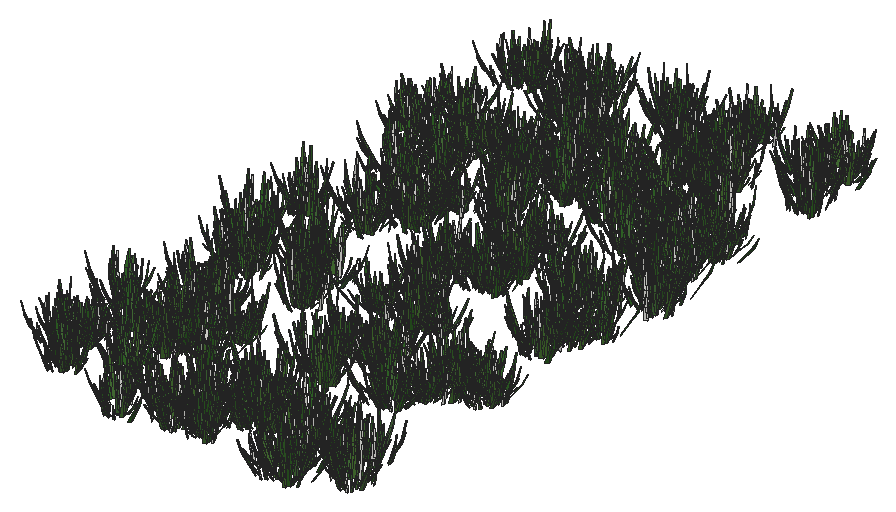
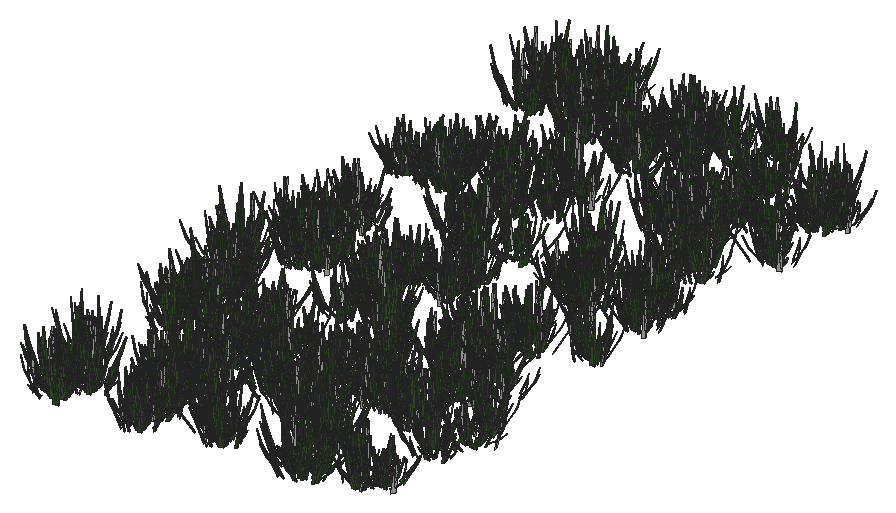
# SketchUp Ruby script. Lengths in inches.
U = 1.inch
M = Sketchup.active_model
def pt(a) = Geom::Point3d.new(a.map { |v| v * U })
def face(e, loops, mat)
  f = e.add_face(loops[0].map { |a| pt(a) })
  loops[1..].each { |l| e.add_face(l.map { |a| pt(a) }).erase! }
  f.material = f.back_material = mat if mat
  f
end
# faces: each face lists its corners as indices into pts; further lists are holes
def faces(e, pts, list, mat = nil) = list.each { |f| face(e, (f[0].is_a?(Array) ? f : [f]).map { |l| l.map { |i| pts[i] } }, mat) }
# xy, xz, yz: faces in a plane at the given z, y or x. An outline is a flat list of corners, or four numbers for a rectangle; further outlines are holes
def ring(l) = l.size == 4 ? [[l[0], l[1]], [l[2], l[1]], [l[2], l[3]], [l[0], l[3]]] : l.each_slice(2).to_a
def flat(e, list, mat, &to3) = list.each { |f| face(e, (f[0].is_a?(Array) ? f : [f]).map { |l| ring(l).map { |u, v| to3.(u, v) } }, mat) }
def xy(e, z, list, mat = nil) = flat(e, list, mat) { |x, y| [x, y, z] }
def xz(e, y, list, mat = nil) = flat(e, list, mat) { |x, z| [x, y, z] }
def yz(e, x, list, mat = nil) = flat(e, list, mat) { |y, z| [x, y, z] }
def lines(e, pts, list) = list.each { |a, b| e.add_line(pt(pts[a]), pt(pts[b])) }
# prism: a flat outline (further loops are holes) pulled along v
def prism(e, loops, v, mat = nil)
  f = face(e, loops, mat); d = Geom::Vector3d.new(v.map { |x| x * U })
  f.pushpull(f.normal.samedirection?(d) ? d.length : -d.length)
end
def box(e, o, s, mat = nil) = prism(e, [[o, [o[0] + s[0], o[1], o[2]], [o[0] + s[0], o[1] + s[1], o[2]], [o[0], o[1] + s[1], o[2]]]], [0, 0, s[2]], mat)
def at(x, y, z, deg = 0) = Geom::Transformation.translation(pt([x, y, z])) * Geom::Transformation.rotation(ORIGIN, Z_AXIS, deg.degrees)
def axes(o, x, y, z) = Geom::Transformation.new([*x, 0, *y, 0, *z, 0, *pt(o).to_a, 1])
def part(name) = M.definitions.add(name)
# library, detail: a bought-in or finely detailed component or shape, given as its bounding box
def library(name, o, s) = part(name).tap { |d| box(d.entities, o, s) }
def detail(e, o, s) = box(e.add_group.entities, o, s)
def put(e, d, t, mat = nil) = e.add_instance(d, t).tap { |i| i.material = mat if mat }
def group(e, t, mat = nil) = e.add_group.tap { |g| g.transformation = t; g.material = mat if mat }.entities
root = M.entities
M.materials.add("Material1").color = [58, 110, 58]
M.materials.add("Material10").color = [48, 100, 38]
M.materials.add("Material3").color = [68, 110, 58]
M.materials.add("Material4").color = [48, 90, 38]
M.materials.add("Material5").color = [68, 110, 48]
M.materials.add("Material6").color = [48, 90, 48]
M.materials.add("Material8").color = [58, 90, 38]
M.materials.add("Material9").color = [68, 100, 58]
c1 = part("grass00")
p = [[-0.6875,0.15,0],[-0.56,0.08,5.52],[-0.04,0.03,2.76],[0.48,-0.02,0],[0.35,-0.02,5.52],[-0.1,-0.14,5.52],
  [-0.12,0.65,8.37],[-0.42,0.65,8.37]]
faces(c1.entities,p,[[0,1,2,3],[3,2,4],[1,5,2],[5,4,2],[1,6,5],[4,5,6],[7,6,1]])
c2 = part("Group16\#1")
put(c2.entities,c1,axes([1.44,-0.61,-0.01],[0.05352,0.12609,0],[-0.10704,0.04543,0.07239],[0.06664,-0.02828,0.11628]),"Material6")
put(c2.entities,c1,axes([0.76,-0.15,-0.01],[0.04676,0.24062,0],[-0.23162,0.04501,0.06642],[0.0652,-0.01267,0.23595]),"Material3")
put(c2.entities,c1,axes([0.79,0.01,-0.01],[-0.00606,0.34651,0],[-0.34381,-0.00602,0.0432],[0.04319,0.00076,0.34386]))
put(c2.entities,c1,axes([1,0.23,-0.01],[-0.07192,0.31144,0],[-0.28722,-0.06632,0.1236],[0.12043,0.02781,0.29478]),"Material5")
put(c2.entities,c1,axes([1.66,0.77,-0.01],[-0.13828,0.29651,0],[-0.21551,-0.1005,0.22471],[0.20365,0.09498,0.23779]),"Material10")
put(c2.entities,c1,axes([0.6875,0.52,-0.01],[-0.18126,0.24051,0],[-0.22746,-0.17142,0.09788],[0.07817,0.05891,0.28481]),"Material5")
put(c2.entities,c1,axes([0.68,0.78,-0.01],[-0.215,0.18688,0],[-0.12385,-0.14248,0.21334],[0.13995,0.16101,0.18878]),"Material3")
put(c2.entities,c1,axes([0.56,1,-0.01],[-0.13756,0.07624,0],[-0.06159,-0.11112,0.0927],[0.04494,0.08108,0.12705]),"Material5")
put(c2.entities,c1,axes([0.2,0.64,-0.01],[-0.23729,0.07254,0],[-0.05711,-0.18681,0.153],[0.04473,0.14632,0.19535]),"Material10")
put(c2.entities,c1,axes([0.0625,0.72,-0.01],[-0.28874,0.02525,0],[-0.02179,-0.24916,0.14647],[0.01276,0.14591,0.25012]),"Material3")
put(c2.entities,c1,axes([-0.08,0.62,-0.01],[-0.34089,-0.04187,0],[0.03255,-0.26504,0.216],[-0.02633,0.21439,0.26703]),"Material10")
put(c2.entities,c1,axes([-0.34,0.98,-0.01],[-0.14314,-0.0493,0],[0.04397,-0.12769,0.06843],[-0.02228,0.0647,0.13505]),"Material10")
put(c2.entities,c1,axes([-0.87,1.45,-0.01],[-0.23488,-0.14114,0],[0.13761,-0.22901,0.06087],[-0.03135,0.05217,0.26717]))
put(c2.entities,c1,axes([-0.72,0.77,-0.01],[-0.14208,-0.13251,0],[0.07209,-0.0773,0.16301],[-0.11118,0.11922,0.1057]),"Material10")
put(c2.entities,c1,axes([-0.62,0.43,-0.01],[-0.14845,-0.21203,0],[0.18654,-0.13061,0.12304],[-0.10079,0.07057,0.22772]),"Material3")
put(c2.entities,c1,axes([-0.68,0.29,-0.01],[-0.13639,-0.32136,0],[0.31723,-0.13464,0.05579],[-0.05136,0.0218,0.34462]),"Material4")
put(c2.entities,c1,axes([-0.64,0.125,-0.01],[-0.0458,-0.23569,0],[0.22124,-0.043,0.08276],[-0.08124,0.01579,0.22538]),"Material1")
put(c2.entities,c1,axes([-1.6,-0.03,-0.01],[0.00576,-0.32897,0],[0.27526,0.00482,0.18018],[-0.18015,-0.00315,0.2753]),"Material5")
put(c2.entities,c1,axes([-1.36,-0.31,-0.01],[0.05718,-0.24765,0],[0.18172,0.04196,0.17267],[-0.16825,-0.03885,0.1865]),"Material10")
put(c2.entities,c1,axes([-1.54,-0.72,-0.01],[0.06537,-0.14017,0],[0.13555,0.06321,0.03939],[-0.0357,-0.01665,0.14956]))
put(c2.entities,c1,axes([-1.19,-0.9,-0.01],[0.09597,-0.12735,0],[0.11214,0.08451,0.07557],[-0.06035,-0.04548,0.14042]),"Material9")
put(c2.entities,c1,axes([-0.47,-0.54,-0.01],[0.11588,-0.10072,0],[0.0618,0.0711,0.12124],[-0.07953,-0.0915,0.0942]))
put(c2.entities,c1,axes([-0.47,-0.84,-0.01],[0.11927,-0.0661,0],[0.06603,0.11913,0.00646],[-0.00313,-0.00565,0.13621]),"Material5")
put(c2.entities,c1,axes([-0.38,-1.24,-0.01],[0.28037,-0.08571,0],[0.0618,0.20215,0.20315],[-0.05939,-0.19428,0.21139]),"Material9")
put(c2.entities,c1,axes([-0.06,-0.66,-0.01],[0.22719,-0.01987,0],[0.01247,0.14255,0.17758],[-0.01547,-0.17691,0.1431]),"Material8")
put(c2.entities,c1,axes([0.11,-0.89,-0.01],[0.14882,0.01828,0],[-0.01058,0.08611,0.12229],[0.01491,-0.12138,0.08676]),"Material6")
put(c2.entities,c1,axes([0.25,-0.72,-0.01],[0.20481,0.07053,0],[-0.06206,0.18022,0.10291],[0.03351,-0.0973,0.1906]),"Material6")
put(c2.entities,c1,axes([0.85,-1.42,-0.01],[0.16481,0.09904,0],[-0.09472,0.15762,0.05616],[0.02893,-0.04814,0.18389]),"Material5")
put(c2.entities,c1,axes([1.01,-1.09,-0.01],[0.21858,0.20385,0],[-0.17495,0.1876,0.15339],[0.10462,-0.11218,0.25652]),"Material10")
put(c2.entities,c1,axes([1.01,-0.71,-0.01],[0.08733,0.12473,0],[-0.06445,0.04512,0.13037],[0.1068,-0.07477,0.07867]),"Material6")
c3 = part("Group15\#1")
put(c3.entities,c2,at(0,0,0))
c4 = part("3darcstudiotree_grass00\#1")
put(c4.entities,c3,at(0,0,0))
put(root,c4,axes([299.44,103.05,0.25],[0.93913,0.57202,0],[-0.54019,0.61097,-0.01519],[-0.01329,0.01503,1.34969]))
put(root,c4,axes([299.53,110.64,0.25],[1.10058,0.261,0],[-0.28805,0.83679,-0.01128],[-0.00476,0.01382,1.61003]))
put(root,c4,axes([300.52,104.49,0.25],[-0.9392,-0.54137,0],[0.54982,-0.65712,-0.00375],[0.00405,-0.00484,1.82358]))
put(root,c4,axes([299.93,147.66,0.25],[0.46431,0.89389,0],[-1.16621,0.41731,-0.01792],[-0.01737,0.00622,1.34035]))
put(root,c4,axes([300.54,144.8125,0.25],[0.73834,-0.68186,0],[0.67706,0.50505,-0.01288],[0.01631,0.01217,1.54961]))
put(root,c4,axes([300.53,103.35,0.25],[0.71679,0.74501,0],[-0.71323,0.47274,-0.01421],[-0.01715,0.01137,1.40932]))
put(root,c4,axes([301.02,122.21,0.25],[-0.0646,-0.98333,0],[0.90905,-0.04114,-0.01049],[0.0169,-0.00076,1.4693]))
put(root,c4,axes([301.24,151.2,0.25],[-0.89627,-0.50604,0],[0.648,-0.79066,-0.01911],[0.01239,-0.01512,1.32815]))
put(root,c4,axes([301.26,131.3,0.25],[0.71286,-0.77446,0],[0.82334,0.52208,-0.00592],[0.00812,0.00515,1.78738]))
put(root,c4,axes([301.23,125.5,0.25],[1.11911,0.29462,0],[-0.34141,0.8934,-0.00141],[-0.00074,0.00193,1.95289]))
put(root,c4,axes([301.5,157.36,0.25],[1.00744,0.57948,0],[-0.6913,0.82795,-0.01195],[-0.00771,0.00924,1.37528]))
put(root,c4,axes([302.64,116.1,0.25],[-0.51912,-0.87799,0],[1.01268,-0.41248,-0.01008],[0.01256,-0.00511,1.566]))
put(root,c4,axes([302.18,99.9375,0.25],[0.69262,0.55781,0],[-0.64459,0.55138,-0.00683],[-0.00897,0.00768,1.74693]))
put(root,c4,axes([302.68,158.2,0.25],[0.15903,-0.85053,0],[0.92507,0.11916,-0.00401],[0.00771,0.00099,1.82024]))
put(root,c4,axes([302.75,122.15,0.25],[-0.79135,0.83075,0],[-0.79545,-0.52199,-0.0043],[-0.00623,-0.00409,1.8735]))
put(root,c4,axes([302.81,107.06,0.25],[0.98585,0.35764,0],[-0.42278,0.80286,-0.01451],[-0.00881,0.01673,1.59989]))
put(root,c4,axes([303.12,140.61,0.25],[1.26422,0.21833,0],[-0.2641,1.05349,-0.01168],[-0.00256,0.01022,1.39591]))
put(root,c4,axes([303.91,120.59,0.25],[0.5832,0.63351,0],[-0.84564,0.53629,-0.0123],[-0.01469,0.00931,1.59876]))
put(root,c4,axes([305.61,148.46,0.25],[-0.29231,-0.74071,0],[1.21148,-0.32935,-0.01545],[0.01785,-0.00485,1.54954]))
put(root,c4,axes([305.17,111.68,0.25],[-0.10149,1.06077,0],[-1.17045,-0.07715,-0.01448],[-0.01792,-0.00118,1.45727]))
put(root,c4,axes([305.58,133.39,0.25],[-1.00175,0.10113,0],[-0.15478,-1.05623,-0.00408],[-0.00067,-0.00459,1.74968]))
put(root,c4,axes([305.25,146.88,0.25],[-0.29516,0.99433,0],[-1.18202,-0.24172,-0.00818],[-0.0119,-0.00243,1.82396]))
put(root,c4,axes([305.51,143.13,0.25],[0.81075,0.69136,0],[-0.85148,0.68788,-0.004],[-0.00456,0.00369,1.89371]))
put(root,c4,axes([306,137.53,0.25],[-1.13548,0.14887,0],[-0.16361,-0.85972,-0.01239],[-0.00262,-0.01379,1.42361]))
put(root,c4,axes([305.7,115.38,0.25],[-0.33676,0.92684,0],[-1.01936,-0.25516,-0.01363],[-0.01733,-0.00434,1.41312]))
put(root,c4,axes([306.17,125.84,0.25],[0.94821,0.33617,0],[-0.44135,0.85759,-0.00364],[-0.00249,0.00485,1.96053]))
put(root,c4,axes([306.94,124.85,0.25],[-0.71892,-0.83603,0],[0.93762,-0.55545,-0.01802],[0.01713,-0.01015,1.345]))
put(root,c4,axes([306.99,160.35,0.25],[-1.10649,-0.54201,0],[0.48134,-0.67694,-0.01139],[0.00932,-0.01311,1.52439]))
put(root,c4,axes([306.61,107.01,0.25],[-0.5773,0.77336,0],[-0.97603,-0.50192,-0.01218],[-0.0144,-0.0074,1.59607]))
put(root,c4,axes([307.02,132.05,0.25],[-0.1247,-0.96853,0],[0.94656,-0.08396,-0.01446],[0.02434,-0.00216,1.61179]))
put(root,c4,axes([307.11,158.32,0.25],[-1.04123,-0.25726,0],[0.30372,-0.84686,-0.0137],[0.00512,-0.01428,1.39479]))
put(root,c4,axes([307.22,108.23,0.25],[-0.87039,-0.77865,0],[0.86634,-0.66714,-0.01209],[0.0122,-0.0094,1.62724]))
put(root,c4,axes([307.23,110.63,0.25],[-0.70394,-0.735,0],[0.91304,-0.60241,-0.01168],[0.01054,-0.00695,1.34439]))
put(root,c4,axes([306.74,102.4,0.25],[0.57245,0.79834,0],[-0.94085,0.46475,-0.00188],[-0.00278,0.00137,1.87843]))
put(root,c4,axes([307.03,109.33,0.25],[-0.54013,0.76401,0],[-1.08788,-0.52983,-0.01374],[-0.01409,-0.00686,1.50009]))
put(root,c4,axes([307.53,139.82,0.25],[0.41756,-0.9912,0],[1.00844,0.29266,-0.01723],[0.02186,0.00634,1.43549]))
put(root,c4,axes([307.39,112.33,0.25],[0.29806,0.83113,0],[-0.93159,0.23015,-0.00785],[-0.01471,0.00363,1.89978]))
put(root,c4,axes([308.14,155.3,0.25],[-0.84934,-0.67408,0],[0.80316,-0.69715,-0.00934],[0.00872,-0.00757,1.57129]))
put(root,c4,axes([308.42,147.1,0.25],[-0.45296,-0.96589,0],[0.97289,-0.31431,-0.00938],[0.0136,-0.00439,1.62403]))
put(root,c4,axes([308.66,137.03,0.25],[0.67888,-0.49311,0],[0.76615,0.72665,-0.0129],[0.01015,0.00963,1.39029]))
put(root,c4,axes([308.91,158.98,0.25],[-1.08195,-0.06614,0],[0.08655,-0.97526,-0.00991],[0.00105,-0.01181,1.69565]))
put(root,c4,axes([308.48,122.28,0.25],[0.67443,0.49943,0],[-0.63457,0.59034,-0.00625],[-0.00755,0.00702,1.72796]))
put(root,c4,axes([309.08,134.5625,0.25],[-0.01664,-0.80699,0],[0.90347,-0.01284,-0.01279],[0.02341,-0.00033,1.65408]))
put(root,c4,axes([309.63,135.52,0.25],[0.00251,-0.99814,0],[1.04954,0.00182,-0.00952],[0.01317,0.00002,1.45276]))
put(root,c4,axes([309.81,153.6875,0.25],[-0.99254,0.21588,0],[-0.25474,-0.80685,-0.00505],[-0.00222,-0.00702,1.74136]))
put(root,c4,axes([309.72,97.17,0.25],[0.88425,-0.78592,0],[0.69052,0.53522,-0.01281],[0.01552,0.01203,1.56626]))
put(root,c4,axes([310.125,112.04,0.25],[-0.4425,-0.69128,0],[1.00597,-0.44361,-0.00698],[0.01022,-0.00451,1.8873]))
put(root,c4,axes([309.72,108.14,0.25],[1.29469,0.00807,0],[-0.00908,1.00371,-0.012],[-0.00013,0.01406,1.70791]))
put(root,c4,axes([310.04,147.6875,0.25],[0.81675,-0.32804,0],[0.42812,0.73432,-0.0104],[0.00662,0.01135,1.43546]))
put(root,c4,axes([309.85,123.82,0.25],[0.13367,0.91551,0],[-1.25012,0.12574,-0.01569],[-0.01838,0.00185,1.48562]))
put(root,c4,axes([310.49,119.4,0.25],[-0.44803,-0.74546,0],[0.92789,-0.38418,-0.00448],[0.00739,-0.00306,1.90991]))
put(root,c4,axes([310.5,138.89,0.25],[-0.92847,-0.18202,0],[0.22811,-0.80158,-0.01801],[0.00557,-0.01958,1.33554]))
put(root,c4,axes([311.33,145.75,0.25],[1.0153,0.11546,0],[-0.1331,0.80633,-0.00884],[-0.00231,0.01402,1.89082]))
put(root,c4,axes([312.07,153.96,0.25],[-0.39516,-0.73082,0],[1.07318,-0.39975,-0.01184],[0.01449,-0.0054,1.57815]))
put(root,c4,axes([312.12,99.8,0.25],[-0.92074,0.49277,0],[-0.52985,-0.68204,-0.01497],[-0.01213,-0.01561,1.4615]))
put(root,c4,axes([312.85,143.85,0.25],[1.09226,-0.42803,0],[0.40892,0.71887,-0.01833],[0.01093,0.01921,1.33779]))
put(root,c4,axes([312.98,149.53,0.25],[1.09823,-0.329,0],[0.37782,0.86885,-0.00463],[0.00252,0.0058,1.7876]))
put(root,c4,axes([312.84,141.85,0.25],[0.33201,0.74072,0],[-1.14012,0.35205,-0.01219],[-0.01224,0.00378,1.30286]))
put(root,c4,axes([313.5625,153.37,0.25],[0.00999,-0.7606,0],[0.96279,0.00871,-0.01263],[0.02232,0.0002,1.70174]))
put(root,c4,axes([314.49,103.04,0.25],[-0.87537,-0.29995,0],[0.36104,-0.72586,-0.01181],[0.00826,-0.0166,1.73426]))
put(root,c4,axes([314.62,102.48,0.25],[0.05871,-0.9503,0],[0.99058,0.04216,-0.01161],[0.0169,0.00072,1.44612]))
put(root,c4,axes([314.32,147.47,0.25],[0.18128,0.97546,0],[-0.98811,0.1265,-0.0058],[-0.01039,0.00133,1.813]))
put(root,c4,axes([314.47,98.3125,0.25],[-0.02897,0.88863,0],[-1.04024,-0.02337,-0.00627],[-0.00978,-0.00022,1.62459]))
put(root,c4,axes([314.63,140.16,0.25],[0.43163,0.66551,0],[-1.03797,0.46376,-0.00648],[-0.00814,0.00364,1.68262]))
put(root,c4,axes([315.26,160.02,0.25],[-0.62972,-0.67404,0],[0.72136,-0.46427,-0.0081],[0.01315,-0.00846,1.87526]))
put(root,c4,axes([315.81,122.57,0.25],[-1.1193,-0.27891,0],[0.34101,-0.94276,-0.01736],[0.00563,-0.01556,1.33702]))
put(root,c4,axes([315.95,100.3,0.25],[-0.82466,-0.67311,0],[0.63771,-0.53823,-0.00764],[0.01069,-0.00902,1.81511]))
put(root,c4,axes([315.96,127.25,0.25],[0.07009,-0.92523,0],[1.03091,0.0538,-0.00515],[0.00872,0.00046,1.75106]))
put(root,c4,axes([315.6875,130.99,0.25],[0.87895,-0.24312,0],[0.35974,0.89596,-0.01535],[0.00664,0.01655,1.5577]))
put(root,c4,axes([316.5,129.89,0.25],[-0.86169,0.23861,0],[-0.30877,-0.76815,-0.01591],[-0.00758,-0.01885,1.46774]))
put(root,c4,axes([316.12,145.21,0.25],[0.84611,0.67014,0],[-0.75348,0.65537,-0.00767],[-0.00889,0.00773,1.8325]))
put(root,c4,axes([316.49,99.65,0.25],[1.02075,-0.0635,0],[0.09548,1.05728,-0.00347],[0.00039,0.00434,1.92949]))
put(root,c4,axes([316.46,158.93,0.25],[1.06818,0.41298,0],[-0.42279,0.75336,-0.0112],[-0.00742,0.01323,1.5714]))
put(root,c4,axes([317.33,149.63,0.25],[0.28495,-0.98406,0],[0.98346,0.19618,-0.00397],[0.007,0.0014,1.83602]))
put(root,c4,axes([317.24,98.42,0.25],[-0.75911,0.72552,0],[-0.71552,-0.51575,-0.01448],[-0.01615,-0.01164,1.39954]))
put(root,c4,axes([317.41,105.58,0.25],[-0.84314,0.75204,0],[-0.91151,-0.704,-0.01383],[-0.01208,-0.00933,1.48532]))
put(root,c4,axes([317.2,151.16,0.25],[0.55593,0.87237,0],[-1.05932,0.46506,-0.01033],[-0.01163,0.00511,1.52631]))
put(root,c4,axes([317.28,112.16,0.25],[1.07243,0.33872,0],[-0.38469,0.83907,-0.01203],[-0.00637,0.01389,1.60927]))
put(root,c4,axes([317.47,136.79,0.25],[-0.53911,0.88923,0],[-1.11267,-0.46471,-0.00338],[-0.00443,-0.00185,1.82725]))
put(root,c4,axes([317.93,125.78,0.25],[-0.84538,-0.30754,0],[0.48939,-0.92675,-0.00176],[0.00113,-0.00214,1.95594]))
put(root,c4,axes([318.03,115.59,0.25],[-0.76406,-0.39576,0],[0.60304,-0.80204,-0.00523],[0.00453,-0.00602,1.86317]))
put(root,c4,axes([317.89,136.2,0.25],[-0.97628,0.3117,0],[-0.33143,-0.71513,-0.01112],[-0.00736,-0.01588,1.70172]))
put(root,c4,axes([319.24,156.42,0.25],[-0.27339,-0.82009,0],[0.86924,-0.19963,-0.0133],[0.02074,-0.00476,1.45899]))
put(root,c4,axes([319.33,122.44,0.25],[-0.01304,-0.82256,0],[1.2333,-0.01347,-0.00745],[0.01173,-0.00013,1.94284]))
put(root,c4,axes([319.39,111,0.25],[0.14472,-0.85297,0],[1.21588,0.14212,-0.00524],[0.00833,0.00097,1.97007]))
put(root,c4,axes([318.92,104.91,0.25],[0.44359,0.66194,0],[-0.79665,0.36778,-0.00131],[-0.00244,0.00113,1.9458]))
put(root,c4,axes([318.96,101.69,0.25],[0.95442,0.55135,0],[-0.6122,0.73006,-0.01513],[-0.01155,0.01377,1.43215]))
put(root,c4,axes([319.58,135.62,0.25],[0.06455,-0.99936,0],[1.28881,0.05734,-0.00697],[0.01022,0.00045,1.89407]))
put(root,c4,axes([319.76,148.36,0.25],[0.90377,0.25855,0],[-0.29349,0.70676,-0.01199],[-0.00572,0.01377,1.31812]))
put(root,c4,axes([319.79,130.6,0.25],[0.92626,0.72851,0],[-0.74994,0.65687,-0.00751],[-0.0086,0.00753,1.8142]))
put(root,c4,axes([320.53,102.41,0.25],[0.11809,-0.96094,0],[1.08149,0.09155,-0.00761],[0.01352,0.00114,1.94156]))
put(root,c4,axes([320.54,133.79,0.25],[0.27551,-0.92727,0],[1.04934,0.21478,-0.00763],[0.01254,0.00257,1.82848]))
put(root,c4,axes([320.71,152.81,0.25],[0.32298,-0.93857,0],[0.99642,0.23621,-0.01145],[0.01514,0.00359,1.42532]))
put(root,c4,axes([320.69,144.83,0.25],[0.58912,-0.58857,0],[0.94383,0.65081,-0.00974],[0.00989,0.00682,1.619]))
put(root,c4,axes([320.8,138.17,0.25],[-0.97679,-0.07818,0],[0.11609,-0.9992,-0.0118],[0.00126,-0.01081,1.34216]))
put(root,c4,axes([320.61,130.52,0.25],[0.92322,0.09717,0],[-0.13089,0.85675,-0.01144],[-0.00235,0.0154,1.7012]))
put(root,c4,axes([321.08,117.55,0.25],[-0.85569,-0.54089,0],[0.64567,-0.70369,-0.01582],[0.01236,-0.01347,1.37394]))
put(root,c4,axes([321.35,154.41,0.25],[-0.62551,-0.56163,0],[0.75996,-0.58308,-0.01026],[0.0126,-0.00967,1.73127]))
put(root,c4,axes([321.76,115.47,0.25],[-0.66763,-0.82572,0],[0.84119,-0.46855,-0.00883],[0.01378,-0.00767,1.90461]))
put(root,c4,axes([321.83,122.54,0.25],[-1.11703,0.06425,0],[-0.06251,-0.74858,-0.01842],[-0.0019,-0.02274,1.34789]))
put(root,c4,axes([321.95,162.05,0.25],[-0.56245,-0.73578,0],[0.81845,-0.431,-0.00968],[0.01463,-0.0077,1.73508]))
put(root,c4,axes([322,159.58,0.25],[-0.16939,-0.77094,0],[1.23948,-0.18761,-0.01194],[0.01483,-0.00225,1.59034]))
put(root,c4,axes([322.03,154.41,0.25],[-0.84925,0.61724,0],[-0.65288,-0.61883,-0.00238],[-0.00301,-0.00286,1.90825]))
put(root,c4,axes([321.96,158.22,0.25],[0.07897,0.94143,0],[-1.01027,0.05838,-0.01352],[-0.01996,0.00115,1.49862]))
put(root,c4,axes([322.42,157.43,0.25],[-0.22075,0.89909,0],[-1.14091,-0.19298,-0.00834],[-0.01214,-0.00205,1.72954]))
put(root,c4,axes([322.53,149.54,0.25],[0.2955,0.86219,0],[-1.20866,0.28537,-0.01266],[-0.01662,0.00392,1.71446]))
put(root,c4,axes([323.98,145.91,0.25],[-0.76953,-0.43703,0],[0.59686,-0.724,-0.01797],[0.01315,-0.01595,1.36964]))
put(root,c4,axes([324.01,104.22,0.25],[-1.21787,0.01808,0],[-0.02029,-0.94162,-0.01042],[-0.0003,-0.01388,1.82123]))
put(root,c4,axes([323.67,103.51,0.25],[0.97049,0.22996,0],[-0.32953,0.95806,-0.00872],[-0.00302,0.00879,1.51538]))
put(root,c4,axes([324.02,155.92,0.25],[0.5621,-0.66071,0],[0.83318,0.48831,-0.00946],[0.01224,0.00717,1.61646]))
put(root,c4,axes([324.94,152.35,0.25],[-0.96297,-0.35751,0],[0.39226,-0.72787,-0.00732],[0.00523,-0.0097,1.68082]))
put(root,c4,axes([324.875,141.9,0.25],[1.00018,0.60209,0],[-0.57698,0.6603,-0.01189],[-0.01068,0.01222,1.50367]))
put(root,c4,axes([324.95,145.94,0.25],[0.94034,0.59141,0],[-0.70983,0.77751,-0.0181],[-0.01253,0.01373,1.34745]))
put(root,c4,axes([325.05,155.14,0.25],[0.23134,0.88526,0],[-0.88217,0.15881,-0.00976],[-0.01718,0.00309,1.62508]))
put(root,c4,axes([325.15,99.24,0.25],[0.89979,0.12113,0],[-0.14763,0.75549,-0.01255],[-0.00356,0.01824,1.63564]))
put(root,c4,axes([325.48,111.27,0.25],[1.12224,0.404,0],[-0.42439,0.81212,-0.01845],[-0.00928,0.01775,1.34771]))
put(root,c4,axes([325.49,97.22,0.25],[0.53454,0.92788,0],[-1.05185,0.41745,-0.01048],[-0.01143,0.00454,1.40926]))
put(root,c4,axes([325.75,111.87,0.25],[-0.00829,1.04332,0],[-1.23748,-0.00677,-0.01347],[-0.01585,-0.00009,1.45625]))
put(root,c4,axes([326.55,147.66,0.25],[-1.12616,-0.21804,0],[0.21083,-0.75017,-0.01564],[0.00524,-0.01866,1.3694]))
put(root,c4,axes([326.36,99.52,0.25],[0.88189,-0.51067,0],[0.56689,0.67442,-0.00731],[0.0076,0.00905,1.80073]))
put(root,c4,axes([327.28,117.37,0.25],[-0.92255,-0.58796,0],[0.66864,-0.72275,-0.00705],[0.00719,-0.00777,1.8369]))
put(root,c4,axes([326.83,97.17,0.25],[1.17981,-0.09399,0],[0.11695,1.01138,-0.01064],[0.00147,0.01275,1.77558]))
put(root,c4,axes([326.78,132.24,0.25],[0.39802,0.8656,0],[-1.12444,0.35618,-0.00597],[-0.00844,0.00267,1.82255]))
put(root,c4,axes([327.41,113.76,0.25],[-0.49445,-0.71053,0],[0.86798,-0.41611,-0.00817],[0.01098,-0.00526,1.55447]))
put(root,c4,axes([327.15,133.34,0.25],[0.89853,0.47239,0],[-0.67289,0.88172,-0.01012],[-0.00683,0.00895,1.58691]))
put(root,c4,axes([328.11,101.63,0.25],[-0.89518,-0.29599,0],[0.45769,-0.95359,-0.00121],[0.0007,-0.00145,1.92636]))
put(root,c4,axes([328.16,115.05,0.25],[-0.8343,0.51207,0],[-0.65921,-0.7399,-0.01371],[-0.00966,-0.01084,1.31321]))
put(root,c4,axes([328.03,126.26,0.25],[0.9149,-0.00797,0],[0.01111,0.87844,-0.01029],[0.00014,0.01121,1.389]))
put(root,c4,axes([328.375,144.67,0.25],[0.44849,-0.96319,0],[1.03945,0.33343,-0.011],[0.01369,0.00439,1.48653]))
put(root,c4,axes([328.14,116.92,0.25],[-0.6013,0.76609,0],[-1.08686,-0.58768,-0.00953],[-0.00909,-0.00491,1.47621]))
put(root,c4,axes([328.77,133.89,0.25],[-0.44008,-0.65891,0],[1.08244,-0.49804,-0.00731],[0.01021,-0.0047,1.97847]))
put(root,c4,axes([328.77,159.74,0.25],[-0.70861,-0.76158,0],[0.85718,-0.54945,-0.00917],[0.01075,-0.00689,1.60374]))
put(root,c4,axes([329.84,124.91,0.25],[0.46887,-0.75145,0],[0.96751,0.41587,-0.01075],[0.01305,0.00561,1.48923]))
put(root,c4,axes([329.93,144.78,0.25],[-1.04523,0.09129,0],[-0.13594,-1.07222,-0.00853],[-0.00119,-0.00939,1.7318]))
put(root,c4,axes([330.0625,103.44,0.25],[-1.14276,-0.11114,0],[0.11042,-0.78217,-0.00847],[0.0019,-0.01345,1.82708]))
put(root,c4,axes([330.2,140.87,0.25],[-1.08116,-0.16646,0],[0.20451,-0.91504,-0.00704],[0.00213,-0.00955,1.86241]))
put(root,c4,axes([329.82,148.18,0.25],[-0.23539,0.96825,0],[-0.9627,-0.16123,-0.00527],[-0.01009,-0.00169,1.91768]))
put(root,c4,axes([329.91,139.88,0.25],[0.49432,0.64735,0],[-1.07538,0.5657,-0.01772],[-0.01621,0.00852,1.37883]))
put(root,c4,axes([330.04,126.97,0.25],[0.71628,0.4961,0],[-0.59469,0.59151,-0.00812],[-0.00905,0.009,1.6158]))
put(root,c4,axes([330.21,162.04,0.25],[-0.1898,0.98322,0],[-1.1812,-0.15708,-0.01053],[-0.01363,-0.00181,1.56894]))
put(root,c4,axes([330.11,128.02,0.25],[1.04665,0.61401,0],[-0.70968,0.8334,-0.0169],[-0.01152,0.01352,1.45184]))
put(root,c4,axes([330.4,141.9,0.25],[-0.67258,0.71766,0],[-0.95462,-0.61632,-0.01031],[-0.01122,-0.00724,1.66779]))
put(root,c4,axes([330.93,161.38,0.25],[0.88299,-0.7174,0],[0.83563,0.70853,-0.00616],[0.00598,0.00507,1.65812]))
put(root,c4,axes([330.97,145.88,0.25],[1.0501,-0.37252,0],[0.41222,0.8005,-0.01454],[0.0071,0.01379,1.30369]))
put(root,c4,axes([331.23,157.65,0.25],[-0.9246,0.0543,0],[-0.08232,-0.96561,-0.01026],[-0.00106,-0.01239,1.70108]))
put(root,c4,axes([331.26,117.2,0.25],[-0.68179,0.76304,0],[-0.87492,-0.53855,-0.0152],[-0.0148,-0.00911,1.3203]))
put(root,c4,axes([331.24,116.3,0.25],[0.24905,1.01065,0],[-1.04541,0.17747,-0.01369],[-0.01763,0.00299,1.40267]))
put(root,c4,axes([331.4,99.55,0.25],[0.07611,0.94919,0],[-1.05595,0.05833,-0.01024],[-0.01758,0.00097,1.82096]))
put(root,c4,axes([331.63,129.96,0.25],[1.01939,0.24913,0],[-0.28884,0.8142,-0.01058],[-0.00449,0.01265,1.53588]))
put(root,c4,axes([331.76,155.75,0.25],[0.88087,0.19943,0],[-0.27571,0.83893,-0.00322],[-0.00161,0.0049,1.99197]))
put(root,c4,axes([331.86,138.03,0.25],[1.2064,0.17215,0],[-0.20113,0.97099,-0.00744],[-0.00195,0.00942,1.83611]))
put(root,c4,axes([332.6,135.58,0.25],[-0.98589,0.18273,0],[-0.24933,-0.92673,-0.00123],[-0.00047,-0.00173,1.99006]))
